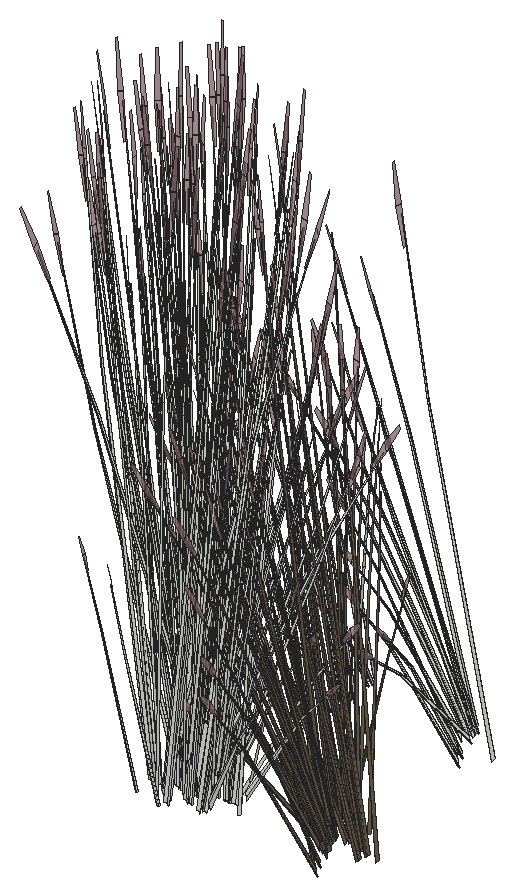
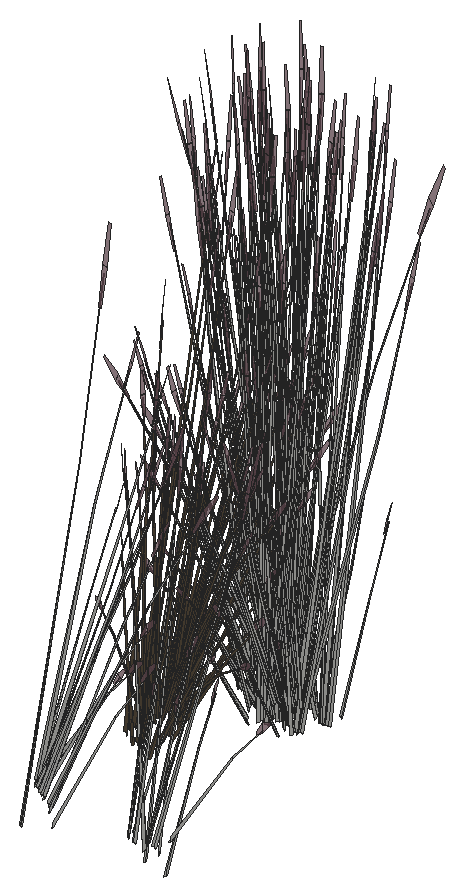
# SketchUp Ruby script. Lengths in inches.
U = 1.inch
M = Sketchup.active_model
def pt(a) = Geom::Point3d.new(a.map { |v| v * U })
def face(e, loops, mat)
  f = e.add_face(loops[0].map { |a| pt(a) })
  loops[1..].each { |l| e.add_face(l.map { |a| pt(a) }).erase! }
  f.material = f.back_material = mat if mat
  f
end
# faces: each face lists its corners as indices into pts; further lists are holes
def faces(e, pts, list, mat = nil) = list.each { |f| face(e, (f[0].is_a?(Array) ? f : [f]).map { |l| l.map { |i| pts[i] } }, mat) }
# xy, xz, yz: faces in a plane at the given z, y or x. An outline is a flat list of corners, or four numbers for a rectangle; further outlines are holes
def ring(l) = l.size == 4 ? [[l[0], l[1]], [l[2], l[1]], [l[2], l[3]], [l[0], l[3]]] : l.each_slice(2).to_a
def flat(e, list, mat, &to3) = list.each { |f| face(e, (f[0].is_a?(Array) ? f : [f]).map { |l| ring(l).map { |u, v| to3.(u, v) } }, mat) }
def xy(e, z, list, mat = nil) = flat(e, list, mat) { |x, y| [x, y, z] }
def xz(e, y, list, mat = nil) = flat(e, list, mat) { |x, z| [x, y, z] }
def yz(e, x, list, mat = nil) = flat(e, list, mat) { |y, z| [x, y, z] }
def lines(e, pts, list) = list.each { |a, b| e.add_line(pt(pts[a]), pt(pts[b])) }
# prism: a flat outline (further loops are holes) pulled along v
def prism(e, loops, v, mat = nil)
  f = face(e, loops, mat); d = Geom::Vector3d.new(v.map { |x| x * U })
  f.pushpull(f.normal.samedirection?(d) ? d.length : -d.length)
end
def box(e, o, s, mat = nil) = prism(e, [[o, [o[0] + s[0], o[1], o[2]], [o[0] + s[0], o[1] + s[1], o[2]], [o[0], o[1] + s[1], o[2]]]], [0, 0, s[2]], mat)
def at(x, y, z, deg = 0) = Geom::Transformation.translation(pt([x, y, z])) * Geom::Transformation.rotation(ORIGIN, Z_AXIS, deg.degrees)
def axes(o, x, y, z) = Geom::Transformation.new([*x, 0, *y, 0, *z, 0, *pt(o).to_a, 1])
def part(name) = M.definitions.add(name)
# library, detail: a bought-in or finely detailed component or shape, given as its bounding box
def library(name, o, s) = part(name).tap { |d| box(d.entities, o, s) }
def detail(e, o, s) = box(e.add_group.entities, o, s)
def put(e, d, t, mat = nil) = e.add_instance(d, t).tap { |i| i.material = mat if mat }
def group(e, t, mat = nil) = e.add_group.tap { |g| g.transformation = t; g.material = mat if mat }.entities
root = M.entities
M.materials.add("Forest_Floor_01_1K").color = [106, 91, 72]
M.materials.add("LightPink_Translucent").color = [144, 107, 117]
M.materials["LightPink_Translucent"].alpha = 0.75
c1 = part("blade")
p = [[2.15,0.21,22],[0,0.17,0],[0.09,0.45,0],[2.18,0.31,22],[2.29,0.31,22],[0.38,0.45,0],
  [2.48,0.24,33],[2.49,0.24,33],[2.48,0.22,33]]
faces(c1.entities,p,[[0,1,2,3],[4,5,2,3],[6,3,4,7],[8,0,3,6]])
c2 = part("seeds")
p = [[0.3,-0.1,1.38],[-0.01,-0.03,1.59],[-0.01,-0.03,0.03],[0.14,-0.07,-0.07],[0.29,-0.03,3],[0.15,0.01,3.11]]
faces(c2.entities,p,[[0,1,2,3],[1,0,4,5]],"LightPink_Translucent")
c3 = part("blade with seeds")
put(c3.entities,c1,at(0,0,0))
put(c3.entities,c2,axes([2.4,0.25,30.99],[1.5799,-0.05474,1.17369],[-0.12525,1.92788,0.29478],[-0.07173,-0.02425,1.56792]))
put(root,c3,axes([495.47,122.05,4.86],[-0.79037,-0.10018,-0.62353],[0.16679,-0.61794,-0.16365],[-0.23587,-0.07488,1.37633]))
put(root,c3,axes([492.67,142.88,3.91],[-0.11621,-0.08567,1.74944],[-0.77555,0.05431,-0.27667],[-0.12378,-0.20491,0.14031]))
put(root,c3,axes([494.4375,123.22,4.82],[-0.7111,-0.30552,-0.49651],[0.42504,-0.54784,0],[-0.16196,-0.06958,1.57504]))
put(root,c3,axes([494.87,123.59,5.17],[-0.47504,0.61229,0],[-0.79476,-0.34146,-0.51607],[-0.18101,-0.07777,1.63711]))
put(root,c3,axes([493.21,144.23,3.875],[-0.7469,-0.15318,-0.51099],[0.25601,-0.52518,-0.3958],[-0.06849,-0.21144,0.97773]))
put(root,c3,axes([494,124.48,5.39],[0.23977,-0.09639,1.43002],[0.59198,0.29065,-0.30754],[-0.1762,0.25149,0.61141]))
put(root,c3,axes([493.66,118.98,4.93],[-0.21918,0.49894,-0.03893],[-0.6746,-0.15348,-0.17649],[-0.10242,-0.08161,0.58215]))
put(root,c3,axes([493.48,144.33,4.17],[-0.36264,-0.49684,-0.71045],[0.74649,-0.27689,0.08574],[-0.0848,-0.24006,1.00501]))
put(root,c3,axes([496.37,122.14,5.47],[-0.76714,0.40567,-0.29095],[-0.51013,-0.57321,-0.50002],[-0.18927,-0.05821,1.59708]))
put(root,c3,axes([493.3,121.26,5.17],[-0.95008,0,0],[0,-0.68292,-0.51607],[0,-0.15554,1.63711]))
put(root,c3,axes([494.63,122.99,4.83],[-0.17848,-0.53243,-0.30978],[0.70886,-0.15119,0.30978],[-0.1429,-0.0614,1.38974]))
put(root,c3,axes([494.25,123.55,7.33],[-0.5141,0.32171,-0.35414],[-0.48666,-0.36734,0.4572],[-0.07405,0.18664,0.87481]))
put(root,c3,axes([496.88,122.59,4.86],[-0.51177,0.45928,-0.62353],[-0.63575,-0.41646,-0.16365],[-0.20507,0.11457,1.37633]))
put(root,c3,axes([494.04,121.08,5.13],[-0.70674,0.51372,0.30756],[-0.70717,-0.50832,-0.36492],[-0.02468,-0.14589,1.64885]))
put(root,c3,axes([496.95,122.5,6.125],[0.65659,0.2464,1.51261],[-0.64324,0.53082,0.59816],[-0.28812,-0.31461,1.26806]))
put(root,c3,axes([497.23,122.33,5.27],[-0.74193,-0.49181,-0.25192],[0.6243,-0.55226,0.5513],[-0.19979,0.05753,1.68216]))
put(root,c3,axes([495.88,121.85,5.01],[-0.45644,-0.51287,-0.44739],[0.69137,-0.36116,0.21531],[-0.14771,-0.06346,1.43643]))
put(root,c3,axes([492.85,143.23,0.6875],[-0.12744,0.02202,1.76342],[-0.70477,-0.24781,-0.26939],[0.01183,-0.2067,0.30037]))
put(root,c3,axes([494.59,123.21,8.14],[-0.01977,0.56521,-0.7886],[-0.83252,-0.03796,0.09517],[-0.08786,0.23945,1.11556]))
put(root,c3,axes([494.58,124.8,5.57],[-0.01966,-0.36332,1.1486],[0.49135,0.25914,0.84392],[-0.09663,0.17317,0.25299]))
put(root,c3,axes([493.55,143.91,3.72],[0.22906,-0.4699,-0.35414],[0.66828,0.13705,0.4572],[-0.06128,-0.18919,0.87481]))
put(root,c3,axes([496.86,122.22,5.01],[-0.82508,0.03772,-0.44739],[-0.07462,-0.62614,0.21531],[-0.14771,0.06346,1.43643]))
put(root,c3,axes([495.28,123.27,5.28],[0.7111,0.30552,0.49651],[-0.42504,0.54784,0],[-0.16196,-0.06958,1.57504]))
put(root,c3,axes([494.3125,124.01,6.16],[0.01669,-0.31544,1.54345],[0.75083,0.16661,0.21329],[-0.06506,0.33618,0.72882]))
put(root,c3,axes([495.95,122.15,5.24],[0.20138,-0.72405,-0.23429],[0.95485,0.12621,0.51271],[-0.16685,-0.09999,1.5644]))
put(root,c3,axes([496.3,122.32,5.42],[-0.14658,0.54532,0.1448],[-0.71613,-0.09466,-0.41347],[-0.13033,-0.05599,1.26744]))
put(root,c3,axes([497.72,123.84,4.82],[-0.7111,0.30552,-0.49651],[-0.42504,-0.54784,0],[-0.16196,0.06958,1.57504]))
put(root,c3,axes([493.51,120.79,4.82],[0,-0.61104,-0.49651],[0.85008,0,0],[0,-0.13917,1.57504]))
put(root,c3,axes([493.875,121.36,5.28],[0,0.61104,0.49651],[-0.85008,0,0],[0,-0.13917,1.57504]))
put(root,c3,axes([497.77,123.67,4.99],[-0.46912,-0.61443,-0.05142],[0.79476,-0.34146,0.51607],[-0.19584,0.0585,1.6363]))
put(root,c3,axes([494.76,123.4,7.81],[0.54391,0.41056,-0.5672],[-0.57458,0.35956,-0.43934],[-0.08276,0.2086,1.08528]))
put(root,c3,axes([497.56,123.6,4.83],[-0.70886,-0.15119,-0.30978],[0.17848,-0.53243,0.30978],[-0.1429,0.0614,1.38974]))
put(root,c3,axes([495.73,121.5,5.47],[-0.85568,-0.29155,-0.29095],[0.41201,-0.61537,-0.50002],[-0.02689,-0.15109,1.59708]))
put(root,c3,axes([497.96,121.32,5.64],[-0.02076,-0.57531,1.41272],[0.93937,0.14913,0.59816],[-0.22217,0.31481,1.3335]))
put(root,c3,axes([494.17,124.01,5.625],[0.69024,-0.1082,0.06507],[0.15868,0.43593,-0.86304],[-0.04376,0.22067,0.7736]))
put(root,c3,axes([497.43,122.05,5.47],[0.08854,0.69723,-0.29095],[-0.92215,0.04216,-0.50002],[-0.16238,0.09287,1.59708]))
put(root,c3,axes([495.38,122.81,6.68],[-0.0186,-0.23452,1.71376],[0.80601,0.15558,0.13857],[-0.04985,0.33422,0.73262]))
put(root,c3,axes([493.67,142.91,1.96],[0.09747,0.35631,1.1486],[-0.54071,-0.19735,0.84392],[0.05818,-0.18244,0.25299]))
put(root,c3,axes([493.875,120.81,4.83],[0.53038,-0.38124,-0.30978],[0.53038,0.38124,0.30978],[0,-0.1228,1.38974]))
put(root,c3,axes([496.27,118.34,4.93],[-0.52505,0.35054,-0.03893],[-0.48109,-0.38392,-0.17649],[-0.03387,-0.10878,0.58215]))
put(root,c3,axes([496.0625,121.8,5.16],[0.96033,0.12874,0.45755],[-0.19544,0.7271,0.17955],[-0.14034,-0.07021,1.58856]))
put(root,c3,axes([495.8125,121.67,5.52],[-0.36864,0.55059,0.44739],[-0.76598,-0.26498,-0.21531],[0,-0.12692,1.43643]))
put(root,c3,axes([495.98,143.49,3.9],[-0.07716,0.04667,1.77383],[-0.75601,-0.15746,-0.16761],[-0.02737,-0.20368,0.31391]))
put(root,c3,axes([495.54,122.96,5.27],[0.81646,-0.16218,0.17642],[0.20161,0.60355,0.35086],[-0.07282,-0.08794,1.60407]))
put(root,c3,axes([496.6,123.06,5],[-0.76598,-0.27433,0],[0.36864,-0.57001,0],[0,0,1.62707]))
put(root,c3,axes([498.37,123.74,5.17],[0.47504,0.61229,0],[-0.79476,0.34146,-0.51607],[-0.18101,0.07777,1.63711]))
put(root,c3,axes([494.82,144.625,3.875],[-0.54391,-0.41056,-0.51099],[0.57458,-0.35956,-0.3958],[0.08276,-0.2086,0.97773]))
put(root,c3,axes([497.97,122.99,5.27],[0.21949,-0.60727,0.17642],[0.8032,0.17185,0.35086],[-0.13875,0.00296,1.60407]))
put(root,c3,axes([497.6,122.1875,5.42],[0.56134,0.36712,0.1448],[-0.46823,0.41419,-0.41347],[-0.13033,0.05599,1.26744]))
put(root,c3,axes([497.4,121.74,5.1],[-0.70674,-0.52593,-0.06131],[0.70717,-0.52625,0],[-0.02468,-0.01837,1.75571]))
put(root,c3,axes([497.59,121.92,5.52],[0.82508,-0.03772,0.44739],[0.07462,0.62614,-0.21531],[-0.14771,0.06346,1.43643]))
put(root,c3,axes([494.46,143.9,1.78],[-0.21597,0.12368,1.43002],[-0.64681,-0.21647,-0.30754],[0.1199,-0.26922,0.61141]))
put(root,c3,axes([497.79,123.36,5.13],[0.95122,0.19861,0.30756],[-0.23797,0.7099,-0.36492],[-0.15744,0.08885,1.64885]))
put(root,c3,axes([498.2,123.32,5.28],[0.7111,-0.30552,0.49651],[0.42504,0.54784,0],[-0.16196,0.06958,1.57504]))
put(root,c3,axes([495.98,121.13,5.16],[0.33034,0.68327,0.45755],[-0.94388,0.2376,0.17955],[0.01154,-0.12555,1.58856]))
put(root,c3,axes([495.83,121.04,5.01],[0.36864,-0.55059,-0.44739],[0.76598,0.26498,0.21531],[0,-0.12692,1.43643]))
put(root,c3,axes([496.77,122.82,5],[-0.24791,-0.5268,0],[0.70791,-0.18448,0],[0,0,1.54371]))
put(root,c3,axes([495.87,123.93,4.29],[0.12297,-0.03325,1.76342],[0.73967,0.18301,-0.26939],[0.02163,0.20626,0.30037]))
put(root,c3,axes([496.03,124.12,7.33],[-0.22906,0.4699,-0.35414],[-0.66828,-0.13705,0.4572],[0.06128,0.18919,0.87481]))
put(root,c3,axes([494.99,144.8125,4.17],[0.01977,-0.56521,-0.71045],[0.83252,0.03796,0.08574],[0.08786,-0.23945,1.00501]))
put(root,c3,axes([497.77,121.78,5.01],[-0.36864,0.55059,-0.44739],[-0.76598,-0.26498,0.21531],[0,0.12692,1.43643]))
put(root,c3,axes([499.23,121.45,5.27],[-0.59697,-0.44509,0.17642],[0.60159,-0.4317,0.35086],[-0.06593,0.0909,1.60407]))
put(root,c3,axes([497.17,121.1875,5.01],[0,-0.70701,0],[0.95008,0,0],[0,0,1.79456]))
put(root,c3,axes([496.28,121.32,5.23],[0.8561,0.29616,0.24065],[-0.41201,0.61537,0.50002],[0,-0.14185,1.60543]))
put(root,c3,axes([497.64,121.47,5.09],[0,0.70667,-0.05637],[-0.95008,0,0],[0,0.02221,1.79368]))
put(root,c3,axes([496.01,120.9,5.52],[-0.82508,0.03772,0.44739],[-0.07462,-0.62614,-0.21531],[0.14771,-0.06346,1.43643]))
put(root,c3,axes([495.62,119.83,5.27],[-0.21949,0.60727,0.17642],[-0.8032,-0.17185,0.35086],[0.13875,-0.00296,1.60407]))
put(root,c3,axes([497.1875,122.84,5.09],[0.33034,0.70197,-0.06012],[-0.94388,0.24598,0],[0.01154,0.02451,1.72173]))
put(root,c3,axes([496.15,143.93,3.91],[-0.00733,-0.12161,1.74944],[-0.61946,-0.35147,-0.27667],[0.09577,-0.21306,0.14031]))
put(root,c3,axes([495.23,119.08,5.17],[-0.47504,-0.61229,0],[0.79476,-0.34146,-0.51607],[0.18101,-0.07777,1.63711]))
put(root,c3,axes([496.1,123.69,7.78],[0.36264,0.49684,-0.71045],[-0.74649,0.27689,0.08574],[0.0848,0.24006,1.00501]))
put(root,c3,axes([499.92,121.92,5],[-0.94962,-0.00489,-0.04976],[0,-0.68292,0.49943],[-0.02984,0.15546,1.58352]))
put(root,c3,axes([498.05,119.86,5.27],[-0.81646,0.16218,0.17642],[-0.20161,-0.60355,0.35086],[0.07282,0.08794,1.60407]))
put(root,c3,axes([496.72,120.74,5.16],[-0.62999,0.55453,0.45755],[-0.74845,-0.4895,0.17955],[0.15188,-0.05534,1.58856]))
put(root,c3,axes([497.79,121.62,5.01],[0.53038,0.39469,0],[-0.53038,0.39469,0],[0,0,1.69266]))
put(root,c3,axes([497.78,121.16,5.52],[0.36864,-0.55059,0.44739],[0.76598,0.26498,-0.21531],[0,0.12692,1.43643]))
put(root,c3,axes([497.46,123.07,5],[0.76598,0.27433,0],[-0.36864,0.57001,0],[0,0,1.74954]))
put(root,c3,axes([504.87,143.36,3.07],[0.28223,0.10528,1.71376],[-0.58406,0.44165,0.13857],[-0.36402,-0.19924,0.73262]))
put(root,c3,axes([494.05,144.53,3.07],[-0.14147,0.21002,1.71376],[-0.59349,-0.43464,0.13857],[0.26773,-0.27089,0.73262]))
put(root,c3,axes([506.33,124.92,3.07],[0.31515,-0.01384,1.71376],[-0.20907,0.5998,0.13857],[-0.44912,-0.0371,0.73262]),"Forest_Floor_01_1K")
put(root,c3,axes([496.375,123.79,7.48],[0.7469,0.15318,-0.51099],[-0.25601,0.52518,-0.3958],[0.06849,0.21144,0.97773]))
put(root,c3,axes([497.54,121.02,5.18],[-0.96033,-0.12874,0.49198],[0.19544,-0.7271,0.19306],[0.14034,0.07021,1.70813]))
put(root,c3,axes([499.72,122.02,4.83],[-0.53038,0.38124,-0.30978],[-0.53038,-0.38124,0.30978],[0,0.1228,1.38974]))
put(root,c3,axes([498.2,121.95,4.9],[0.2786,0.55945,-0.69212],[-0.80253,0.20149,-0.18165],[0.03079,0.18945,1.52773]))
put(root,c3,axes([497.8125,121.35,5.01],[0.85008,0,0],[0,0.63259,0],[0,0,1.78407]))
put(root,c3,axes([496.99,120.65,5.52],[-0.45644,-0.51287,0.44739],[0.69137,-0.36116,-0.21531],[0.14771,0.06346,1.43643]))
put(root,c3,axes([496.16,120.77,5.47],[-0.08854,-0.69723,-0.29095],[0.92215,-0.04216,-0.50002],[0.16238,-0.09287,1.59708]))
put(root,c3,axes([498.1,121.28,5.42],[0.70791,-0.1782,0.1448],[0.24791,0.50885,-0.41347],[0,0.11199,1.26744]))
put(root,c3,axes([506.46,125.98,3.07],[0.26363,-0.12925,1.71376],[0.22195,0.59723,0.13857],[-0.41388,0.13498,0.73262]),"Forest_Floor_01_1K")
put(root,c3,axes([497.86,121.32,5.47],[0.85568,0.29155,-0.29095],[-0.41201,0.61537,-0.50002],[0.02689,0.15109,1.59708]))
put(root,c3,axes([505.64,127,1.78],[0.26405,0.05016,1.43002],[0.17019,0.51235,-0.30754],[-0.35868,0.0959,0.61141]),"Forest_Floor_01_1K")
put(root,c3,axes([496.04,119.23,4.83],[0.70886,0.15119,-0.30978],[-0.17848,0.53243,0.30978],[0.1429,-0.0614,1.38974]))
put(root,c3,axes([507.98,125.36,2.53],[0.21597,-0.08839,1.77064],[0.07448,0.61717,0.13857],[-0.4678,0.08189,0.63284]),"Forest_Floor_01_1K")
put(root,c3,axes([499.72,121.46,5.28],[0,-0.61104,0.49651],[0.85008,0,0],[0,0.13917,1.57504]))
put(root,c3,axes([500.08,122.03,4.82],[0,0.61104,-0.49651],[-0.85008,0,0],[0,0.13917,1.57504]))
put(root,c3,axes([495.875,118.99,4.82],[0.7111,-0.30552,-0.49651],[0.42504,0.54784,0],[0.16196,-0.06958,1.57504]))
put(root,c3,axes([496.8,122.71,6.68],[-0.17368,-0.19618,1.71376],[0.80256,-0.16516,0.13857],[0.18139,0.30799,0.73262]))
put(root,c3,axes([497.3,120.5,5.42],[0.14658,-0.54532,0.1448],[0.71613,0.09466,-0.41347],[0.13033,0.05599,1.26744]))
put(root,c3,axes([498.32,119.55,5.28],[-0.7111,-0.30552,0.49651],[0.42504,-0.54784,0],[0.16196,0.06958,1.57504]))
put(root,c3,axes([505.65,125.77,3.91],[-0.12407,0.07933,1.74944],[0.01055,0.57963,-0.27667],[-0.2844,0.07538,0.14031]),"Forest_Floor_01_1K")
put(root,c3,axes([507.27,124.37,4.17],[-0.75952,-0.01471,-0.71045],[0.05101,-0.61953,0.08574],[-0.32177,-0.06538,1.00501]),"Forest_Floor_01_1K")
put(root,c3,axes([506.66,124.52,1.78],[0.14835,0.17012,1.43002],[-0.34183,0.46242,-0.30754],[-0.351,-0.11053,0.61141]),"Forest_Floor_01_1K")
put(root,c3,axes([497.7,122.75,4.99],[0.79769,-0.20732,-0.19198],[0.2803,0.59721,0.00008],[0.08805,-0.02292,1.73897]))
put(root,c3,axes([506.05,125.4375,3.72],[-0.63144,-0.17046,-0.35414],[0.18417,-0.49731,0.4572],[-0.25423,0.0456,0.87481]),"Forest_Floor_01_1K")
put(root,c3,axes([506.93,123.96,3.07],[0.28223,0.10528,1.71376],[-0.58406,0.44165,0.13857],[-0.36402,-0.19924,0.73262]),"Forest_Floor_01_1K")
put(root,c3,axes([504.28,126.36,3.9],[0.09697,0.01639,1.77383],[0.29997,0.53988,-0.16761],[-0.1985,0.1417,0.31391]),"Forest_Floor_01_1K")
put(root,c3,axes([506.49,125.69,3.875],[-0.20584,0.55581,-0.51099],[-0.70573,-0.19051,-0.3958],[-0.28414,0.05097,0.97773]),"Forest_Floor_01_1K")
put(root,c3,axes([497.71,120.97,5.01],[0.45644,0.51287,-0.44739],[-0.69137,0.36116,0.21531],[0.14771,0.06346,1.43643]))
put(root,c3,axes([507.02,124.49,3.875],[-0.55171,0.40476,-0.51099],[-0.48318,-0.42758,-0.3958],[-0.28031,-0.06159,0.97773]),"Forest_Floor_01_1K")
put(root,c3,axes([506.13,125.66,0.6875],[0.01927,0.0963,1.76342],[-0.38846,0.5029,-0.26939],[-0.27592,-0.02535,0.30037]),"Forest_Floor_01_1K")
put(root,c3,axes([499,123.3,5.57],[-0.4278,-0.1757,1.1486],[0.5524,-0.17852,0.84392],[0.14899,0.15122,0.25299]))
put(root,c3,axes([497.48,123.11,5.39],[0.01341,-0.20255,1.43002],[0.64074,-0.22625,-0.30754],[0.1978,0.24243,0.61141]))
put(root,c3,axes([506.76,142.5625,4.62],[-0.50709,0.58578,-0.13619],[-0.73436,-0.33748,-0.75594],[-0.25527,-0.1655,1.14864]))
put(root,c3,axes([506.24,123.36,3.9],[0.05633,0.06098,1.77383],[-0.27155,0.54815,-0.16761],[-0.27501,0.00397,0.31391]),"Forest_Floor_01_1K")
put(root,c3,axes([496.72,120.24,4.86],[0.51177,-0.45928,-0.62353],[0.63575,0.41646,-0.16365],[0.20507,-0.11457,1.37633]))
put(root,c3,axes([505.09,128.07,1.96],[0.31665,-0.27694,1.1486],[0.12495,0.43841,0.84392],[-0.22883,0.0785,0.25299]),"Forest_Floor_01_1K")
put(root,c3,axes([506.54,143.04,4.17],[-0.64788,-0.29534,-0.71045],[0.46044,-0.51755,0.08574],[-0.23473,-0.17635,1.00501]))
put(root,c3,axes([506.24,143.05,3.875],[-0.74975,0.14525,-0.51099],[-0.13115,-0.55007,-0.3958],[-0.20138,-0.15763,0.97773]))
put(root,c3,axes([506.87,122.99,3.91],[-0.16348,-0.00431,1.74944],[-0.52047,0.43131,-0.27667],[-0.2777,-0.08813,0.14031]),"Forest_Floor_01_1K")
put(root,c3,axes([506.2,125.38,3.93],[0.21466,-0.55714,0.48003],[0.70573,0.19051,0.3958],[-0.27753,0.03348,0.9933]),"Forest_Floor_01_1K")
put(root,c3,axes([498.96,119.83,4.83],[0.17848,0.53243,-0.30978],[-0.70886,0.15119,0.30978],[0.1429,0.0614,1.38974]))
put(root,c3,axes([500.3,121.57,5.18],[0.95008,0,0],[0,0.68292,-0.51607],[0,0.15554,1.63711]))
put(root,c3,axes([506.45,125.22,4.23],[0.38229,0.5533,-0.1216],[-0.6785,0.2719,-0.67495],[-0.28593,0.073,1.02557]),"Forest_Floor_01_1K")
put(root,c3,axes([507.3125,124.07,4.23],[-0.04068,0.62141,-0.1216],[-0.77029,-0.01698,-0.67495],[-0.29667,-0.04317,1.02557]),"Forest_Floor_01_1K")
put(root,c3,axes([506.82,124.11,3.72],[-0.43232,-0.38257,-0.35414],[0.49364,-0.36215,0.4572],[-0.25081,-0.0551,0.87481]),"Forest_Floor_01_1K")
put(root,c3,axes([505.27,142.55,0.6875],[-0.0736,0.08049,1.76342],[-0.74378,0.17355,-0.26939],[-0.17968,-0.15788,0.30037]))
put(root,c3,axes([506.15,125.23,3.92],[-0.27906,-0.41663,0.0643],[0.50888,-0.20393,0.50621],[-0.22432,0.04024,0.77189]),"Forest_Floor_01_1K")
put(root,c3,axes([507.43,126.38,3.07],[0.18977,-0.18775,1.71376],[0.47917,0.50677,0.13857],[-0.32866,0.23079,0.73262]),"Forest_Floor_01_1K")
put(root,c3,axes([506.28,126.875,3.72],[-0.66138,0.08733,-0.35414],[-0.17464,-0.49921,0.4572],[-0.18953,0.13408,0.87481]),"Forest_Floor_01_1K")
put(root,c3,axes([497.23,120.68,5.47],[0.76714,-0.40567,-0.29095],[0.51013,0.57321,-0.50002],[0.18927,0.05821,1.59708]))
put(root,c3,axes([499.07,124.1,5.47],[-0.48723,-0.01916,1.0506],[0.32177,-0.40701,0.58006],[0.19248,0.1446,0.8241]))
put(root,c3,axes([505.92,128.36,0.6875],[0.10192,0.06105,1.76342],[0.17281,0.56562,-0.26939],[-0.22588,0.12062,0.30037]),"Forest_Floor_01_1K")
put(root,c3,axes([505.78,125.03,1.96],[0.48508,-0.04372,1.1486],[-0.3077,0.38525,0.84392],[-0.23971,-0.05779,0.25299]),"Forest_Floor_01_1K")
put(root,c3,axes([506.37,126.77,3.93],[-0.18844,-0.56237,0.48003],[0.73919,-0.0976,0.3958],[-0.21785,0.13226,0.9933]),"Forest_Floor_01_1K")
put(root,c3,axes([506.75,123.97,4.29],[0.62747,-0.45094,0.53763],[0.54116,0.47889,0.4433],[-0.29439,-0.08318,1.11249]),"Forest_Floor_01_1K")
put(root,c3,axes([495.29,120.32,4.39],[-0.74787,0.24464,1.28929],[-0.23804,-0.70192,0.50096],[0.45924,0.01168,1.46642]))
put(root,c3,axes([506.22,126.66,3.92],[-0.52161,-0.25698,0.0643],[0.30368,-0.36595,0.50621],[-0.16723,0.11831,0.77189]),"Forest_Floor_01_1K")
put(root,c3,axes([506.57,141.17,3.9],[-0.01417,0.07324,1.77383],[-0.6991,0.2658,-0.16761],[-0.20573,-0.13587,0.31391]))
put(root,c3,axes([507.28,126.84,3.07],[0.14147,-0.21002,1.71376],[0.59349,0.43464,0.13857],[-0.26773,0.27089,0.73262]),"Forest_Floor_01_1K")
put(root,c3,axes([505.82,142.23,1.78],[-0.04601,0.19989,1.43002],[-0.67263,0.16733,-0.30754],[-0.15723,-0.25836,0.61141]))
put(root,c3,axes([498.04,123.54,7.48],[0.74975,-0.14525,-0.51099],[0.13115,0.55007,-0.3958],[0.20138,0.15763,0.97773]))
put(root,c3,axes([506.04,142.75,3.07],[0.17368,0.19618,1.71376],[-0.80256,0.16516,0.13857],[-0.18139,-0.30799,0.73262]))
put(root,c3,axes([498.73,119.23,5.18],[0.47504,-0.61229,0],[0.79476,0.34146,-0.51607],[0.18101,0.07777,1.63711]))
put(root,c3,axes([506.72,125.38,4.24],[0.63144,0.17046,0.35414],[-0.18417,0.49731,-0.4572],[-0.25423,0.0456,0.87481]),"Forest_Floor_01_1K")
put(root,c3,axes([506.32,142.65,3.72],[-0.11735,-0.49217,-0.35414],[0.67083,-0.12996,0.4572],[-0.18018,-0.14104,0.87481]))
put(root,c3,axes([499.16,119.6,4.82],[0.7111,0.30552,-0.49651],[-0.42504,0.54784,0],[0.16196,0.06958,1.57504]))
put(root,c3,axes([506.83,126.93,3.875],[0.19519,0.55794,-0.51099],[-0.73919,0.0976,-0.3958],[-0.21183,0.14986,0.97773]),"Forest_Floor_01_1K")
put(root,c3,axes([499.125,123.95,4.29],[0.05536,-0.08822,1.76342],[0.69692,-0.25981,-0.26939],[0.21129,0.13447,0.30037]))
put(root,c3,axes([507.04,123.96,3.92],[0.03826,-0.46465,0.0643],[0.57772,0.01274,0.50621],[-0.2213,-0.04862,0.77189]),"Forest_Floor_01_1K")
put(root,c3,axes([499.5,120.26,7.48],[-0.19519,-0.55794,-0.51099],[0.73919,-0.0976,-0.3958],[0.21183,-0.14986,0.97773]))
put(root,c3,axes([505.67,127.93,3.91],[-0.01889,0.12092,1.74944],[0.53598,0.42065,-0.27667],[-0.14032,0.19892,0.14031]),"Forest_Floor_01_1K")
put(root,c3,axes([508.67,126.53,1.25],[-0.79037,-0.10018,-0.62353],[0.16679,-0.61794,-0.16365],[-0.23587,-0.07488,1.37633]),"Forest_Floor_01_1K")
put(root,c3,axes([508.81,123.16,4.62],[-0.50709,0.58578,-0.13619],[-0.73436,-0.33748,-0.75594],[-0.25527,-0.1655,1.14864]),"Forest_Floor_01_1K")
put(root,c3,axes([500.8,123.14,6.73],[-0.14542,-0.51365,-0.03492],[0.68734,-0.11809,-0.15832],[0.14353,0.03256,0.52218]))
put(root,c3,axes([507.43,124.3125,4.24],[0.43232,0.38257,0.35414],[-0.49364,0.36215,-0.4572],[-0.25081,-0.0551,0.87481]),"Forest_Floor_01_1K")
put(root,c3,axes([498.125,120.77,4.86],[0.79037,0.10018,-0.62353],[-0.16679,0.61794,-0.16365],[0.23587,0.07488,1.37633]))
put(root,c3,axes([508.59,123.64,4.17],[-0.64788,-0.29534,-0.71045],[0.46044,-0.51755,0.08574],[-0.23473,-0.17635,1.00501]),"Forest_Floor_01_1K")
put(root,c3,axes([508.29,123.65,3.875],[-0.74975,0.14525,-0.51099],[-0.13115,-0.55007,-0.3958],[-0.20138,-0.15763,0.97773]),"Forest_Floor_01_1K")
put(root,c3,axes([501.49,121.14,5.0625],[-0.47106,-0.39072,-0.06488],[0.51591,-0.35801,-0.29416],[0.14618,-0.02521,0.97024]))
put(root,c3,axes([507.64,127.7,1.21],[-0.7111,-0.30552,-0.49651],[0.42504,-0.54784,0],[-0.16196,-0.06958,1.57504]),"Forest_Floor_01_1K")
put(root,c3,axes([500.41,119.15,5.57],[-0.25308,0.31105,1.1486],[-0.21753,-0.4179,0.84392],[0.20902,-0.10472,0.25299]))
put(root,c3,axes([505.58,141.91,1.96],[0.39634,0.21267,1.1486],[-0.57721,0.12784,0.84392],[-0.1235,-0.16344,0.25299]))
put(root,c3,axes([507.32,123.15,0.6875],[-0.0736,0.08049,1.76342],[-0.74378,0.17355,-0.26939],[-0.17968,-0.15788,0.30037]),"Forest_Floor_01_1K")
put(root,c3,axes([506.48,126.53,4.23],[0.70283,0.33692,-0.1216],[-0.40491,0.48793,-0.67495],[-0.19857,0.16961,1.02557]),"Forest_Floor_01_1K")
put(root,c3,axes([508.07,128.07,1.57],[-0.47504,0.61229,0],[-0.79476,-0.34146,-0.51607],[-0.18101,-0.07777,1.63711]),"Forest_Floor_01_1K")
put(root,c3,axes([506.41,142.47,4.29],[0.84639,-0.15705,0.53763],[0.14689,0.61608,0.4433],[-0.19906,-0.18157,1.11249]))
put(root,c3,axes([505.32,128,4.84],[0.67048,0.16311,-0.06488],[-0.20625,0.50201,-0.29416],[-0.10966,0.07622,0.97024]),"Forest_Floor_01_1K")
put(root,c3,axes([497.96,122.1,6.68],[-0.28223,-0.10528,1.71376],[0.58406,-0.44165,0.13857],[0.36402,0.19924,0.73262]))
put(root,c3,axes([506.61,142.6,3.92],[0.34533,-0.38816,0.0643],[0.49176,0.22599,0.50621],[-0.15898,-0.12445,0.77189]))
put(root,c3,axes([506.82,126.58,4.24],[0.66138,-0.08733,0.35414],[0.17464,0.49921,-0.4572],[-0.18953,0.13408,0.87481]),"Forest_Floor_01_1K")
put(root,c3,axes([500.05,120.32,7.33],[0.66138,-0.08733,-0.35414],[0.17464,0.49921,0.4572],[0.18953,-0.13408,0.87481]))
put(root,c3,axes([507.2,128.96,1.78],[0.23977,-0.09639,1.43002],[0.59198,0.29065,-0.30754],[-0.1762,0.25149,0.61141]),"Forest_Floor_01_1K")
put(root,c3,axes([499.52,120.48,7.78],[0.39688,-0.48213,-0.71045],[0.69548,0.34264,0.08574],[0.23697,-0.17468,1.00501]))
put(root,c3,axes([506.86,123.46,1.32],[-0.21918,0.49894,-0.03893],[-0.6746,-0.15348,-0.17649],[-0.10242,-0.08161,0.58215]),"Forest_Floor_01_1K")
put(root,c3,axes([499.51,123.08,7.33],[0.43232,0.38257,-0.35414],[-0.49364,0.36215,0.4572],[0.25081,0.0551,0.87481]))
put(root,c3,axes([508.62,121.77,3.9],[-0.01417,0.07324,1.77383],[-0.6991,0.2658,-0.16761],[-0.20573,-0.13587,0.31391]),"Forest_Floor_01_1K")
put(root,c3,axes([507.36,141.45,3.91],[-0.11621,-0.08567,1.74944],[-0.77555,0.05431,-0.27667],[-0.12378,-0.20491,0.14031]))
put(root,c3,axes([507.87,122.83,1.78],[-0.04601,0.19989,1.43002],[-0.67263,0.16733,-0.30754],[-0.15723,-0.25836,0.61141]),"Forest_Floor_01_1K")
put(root,c3,axes([508.09,123.35,3.07],[0.17368,0.19618,1.71376],[-0.80256,0.16516,0.13857],[-0.18139,-0.30799,0.73262]),"Forest_Floor_01_1K")
put(root,c3,axes([509.57,126.62,1.86],[-0.76714,0.40567,-0.29095],[-0.51013,-0.57321,-0.50002],[-0.18927,-0.05821,1.59708]),"Forest_Floor_01_1K")
put(root,c3,axes([507.45,127.9,3.93],[-0.54105,-0.41691,0.48003],[0.57458,-0.35956,0.3958],[-0.0998,0.1956,0.9933]),"Forest_Floor_01_1K")
put(root,c3,axes([508.37,123.25,3.72],[-0.11735,-0.49217,-0.35414],[0.67083,-0.12996,0.4572],[-0.18018,-0.14104,0.87481]),"Forest_Floor_01_1K")
put(root,c3,axes([506.5,125.74,1.57],[-0.95008,0,0],[0,-0.68292,-0.51607],[0,-0.15554,1.63711]),"Forest_Floor_01_1K")
put(root,c3,axes([507.83,127.47,1.22],[-0.17848,-0.53243,-0.30978],[0.70886,-0.15119,0.30978],[-0.1429,-0.0614,1.38974]),"Forest_Floor_01_1K")
put(root,c3,axes([507.25,127.86,3.92],[-0.62439,-0.02847,0.0643],[0.01712,-0.42991,0.50621],[-0.06534,0.16468,0.77189]),"Forest_Floor_01_1K")
put(root,c3,axes([507.45,128.03,3.72],[-0.5141,0.32171,-0.35414],[-0.48666,-0.36734,0.4572],[-0.07405,0.18664,0.87481]),"Forest_Floor_01_1K")
put(root,c3,axes([499.84,121.5,7.48],[0.20584,-0.55581,-0.51099],[0.70573,0.19051,-0.3958],[0.28414,-0.05097,0.97773]))
put(root,c3,axes([501.62,121.85,5.57],[-0.46945,0.10088,1.1486],[0.22097,-0.4169,0.84392],[0.24904,0.02853,0.25299]))
put(root,c3,axes([510.08,127.07,1.25],[-0.51177,0.45928,-0.62353],[-0.63575,-0.41646,-0.16365],[-0.20507,0.11457,1.37633]),"Forest_Floor_01_1K")
put(root,c3,axes([508.77,123.65,4.24],[0.11735,0.49217,0.35414],[-0.67083,0.12996,-0.4572],[-0.18018,-0.14104,0.87481]),"Forest_Floor_01_1K")
put(root,c3,axes([505.61,129.17,3.9],[0.0862,-0.03689,1.77383],[0.71245,0.24539,-0.16761],[-0.01674,0.20431,0.31391]),"Forest_Floor_01_1K")
put(root,c3,axes([506.5,144.76,1.29],[-0.31203,-0.62659,-0.69835],[0.89884,-0.22566,-0.18329],[-0.03449,-0.21218,1.54149]))
